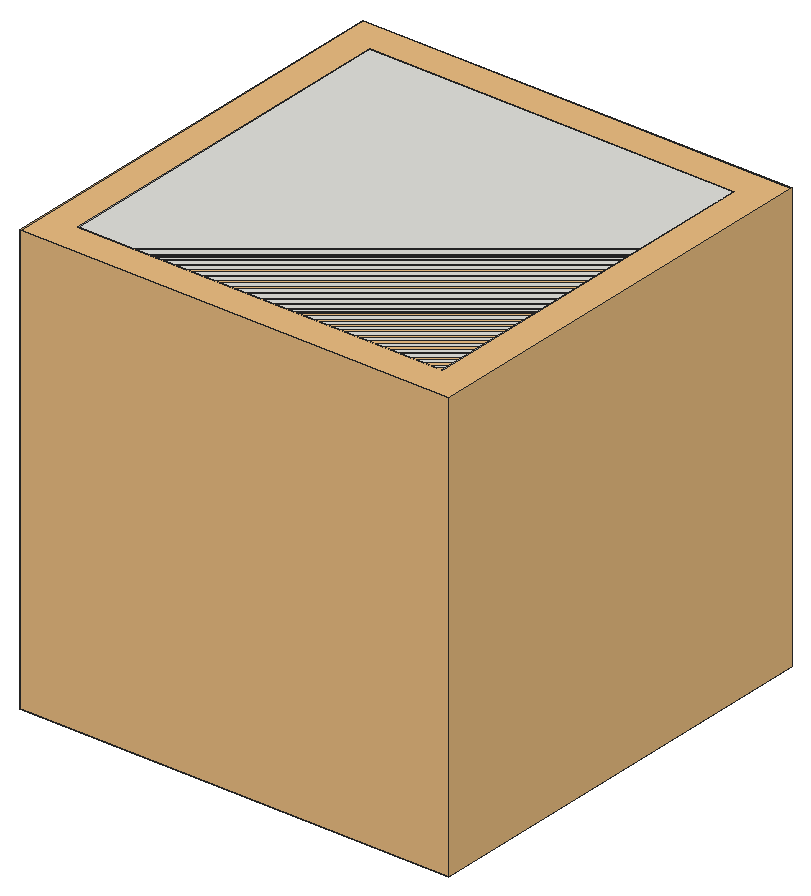
# SketchUp Ruby script. Lengths in inches.
U = 1.inch
M = Sketchup.active_model
def pt(a) = Geom::Point3d.new(a.map { |v| v * U })
def face(e, loops, mat)
  f = e.add_face(loops[0].map { |a| pt(a) })
  loops[1..].each { |l| e.add_face(l.map { |a| pt(a) }).erase! }
  f.material = f.back_material = mat if mat
  f
end
# faces: each face lists its corners as indices into pts; further lists are holes
def faces(e, pts, list, mat = nil) = list.each { |f| face(e, (f[0].is_a?(Array) ? f : [f]).map { |l| l.map { |i| pts[i] } }, mat) }
# xy, xz, yz: faces in a plane at the given z, y or x. An outline is a flat list of corners, or four numbers for a rectangle; further outlines are holes
def ring(l) = l.size == 4 ? [[l[0], l[1]], [l[2], l[1]], [l[2], l[3]], [l[0], l[3]]] : l.each_slice(2).to_a
def flat(e, list, mat, &to3) = list.each { |f| face(e, (f[0].is_a?(Array) ? f : [f]).map { |l| ring(l).map { |u, v| to3.(u, v) } }, mat) }
def xy(e, z, list, mat = nil) = flat(e, list, mat) { |x, y| [x, y, z] }
def xz(e, y, list, mat = nil) = flat(e, list, mat) { |x, z| [x, y, z] }
def yz(e, x, list, mat = nil) = flat(e, list, mat) { |y, z| [x, y, z] }
def lines(e, pts, list) = list.each { |a, b| e.add_line(pt(pts[a]), pt(pts[b])) }
# prism: a flat outline (further loops are holes) pulled along v
def prism(e, loops, v, mat = nil)
  f = face(e, loops, mat); d = Geom::Vector3d.new(v.map { |x| x * U })
  f.pushpull(f.normal.samedirection?(d) ? d.length : -d.length)
end
def box(e, o, s, mat = nil) = prism(e, [[o, [o[0] + s[0], o[1], o[2]], [o[0] + s[0], o[1] + s[1], o[2]], [o[0], o[1] + s[1], o[2]]]], [0, 0, s[2]], mat)
def at(x, y, z, deg = 0) = Geom::Transformation.translation(pt([x, y, z])) * Geom::Transformation.rotation(ORIGIN, Z_AXIS, deg.degrees)
def axes(o, x, y, z) = Geom::Transformation.new([*x, 0, *y, 0, *z, 0, *pt(o).to_a, 1])
def part(name) = M.definitions.add(name)
# library, detail: a bought-in or finely detailed component or shape, given as its bounding box
def library(name, o, s) = part(name).tap { |d| box(d.entities, o, s) }
def detail(e, o, s) = box(e.add_group.entities, o, s)
def put(e, d, t, mat = nil) = e.add_instance(d, t).tap { |i| i.material = mat if mat }
def group(e, t, mat = nil) = e.add_group.tap { |g| g.transformation = t; g.material = mat if mat }.entities
root = M.entities
M.materials.add("Pomeli-edt-511x511").color = [242, 209, 211]
M.materials.add("profumo-muschio-natures-511x511").color = [223, 234, 229]
c1 = library("Round ottoman",[0,0,0],[24.18,24.17,17.98])
c2 = library("Decoração+Banheiro",[28.69,-29.77,58.91],[5.39,6.58,5.91])
c3 = library("skpA613",[-33.11,-37.89,-86.79],[66.22,75.78,173.58])
c4 = library("Potted plant",[0.24,-1.94,0],[14.49,14.49,6.23])
c5 = library("ADORNOS+-+RMLLR",[6.19,-1.3125,-0.22],[15.35,11.9,12.07])
c6 = library("Toiletry bottle \#2",[0,0,0],[4.22,2.62,10.91])
c7 = library("Toiletry bottle \#3",[0,0,0],[4.22,2.62,10.91])
c8 = library("Toiletry bottle",[0,0,0],[3.45,3.45,11.12])
c9 = part("Component\#12")
xy(c9.entities,0,[[0,0,3.21,3.15]],"profumo-muschio-natures-511x511")
xy(c9.entities,9.32,[[0,0,3.21,3.15]])
xz(c9.entities,0,[[0,0,3.21,9.32]],"profumo-muschio-natures-511x511")
xz(c9.entities,3.15,[[0,0,3.21,9.32]])
yz(c9.entities,0,[[0,0,3.15,9.32]])
yz(c9.entities,3.21,[[0,0,3.15,9.32]])
c10 = library("Toiletry bottle \#1",[0,0,0],[3.45,3.45,11.12])
c11 = part("Component\#17")
xy(c11.entities,0,[[0,0,3.21,3.15]],"profumo-muschio-natures-511x511")
xy(c11.entities,9.32,[[0,0,3.21,3.15]])
xz(c11.entities,0,[[0,0,3.21,9.32]],"Pomeli-edt-511x511")
xz(c11.entities,3.15,[[0,0,3.21,9.32]])
yz(c11.entities,0,[[0,0,3.15,9.32]])
yz(c11.entities,3.21,[[0,0,3.15,9.32]])
c12 = library("Plant",[-15.17,-14.95,0],[35.27,31.45,46.14])
c13 = library("FILE+KEEPER",[308.125,87.4375,-0.08],[14,9.09,13.53])
c14 = library("Abstract sculpture",[0,0.06,0],[4.875,4.76,11.74])
c15 = library("Man+sculpture",[-5.14,-9.4,0],[7.87,19.56,27.58])
c16 = library("Group\#6",[0,0,0],[23.16,7,38.98])
c17 = library("Group\#5",[0,0,0],[23.16,7,38.98])
p = [[9,42.4,38],[9,42.4,39.47],[9,90.73,52.9],[9,90.73,52.9],[9,90.73,92.5],[9,90.73,92.5],
  [9,90.73,66.1],[9,90.73,66.1],[9,90.73,79.3],[9,90.73,79.3],[9,42.4,57.58],[9,42.4,106.96],
  [7.875,42.4,39.47],[9,18.02,39.47],[8.9375,18.02,39.47],[10,88.73,25.62],[21,88.73,25.62],[10,90.73,25.62],
  [21,90.73,25.62]]
lines(root,p,[[0,1],[2,3],[4,5],[6,7],[8,9],[10,11],[1,12],[13,14],[15,16],[17,18]])
detail(root,[0,0,0],[120,120,120])
put(root,c1,at(11.49,47.78,2))
put(root,c2,axes([-13.4,59.45,-37.71],[1,0,0],[0,1.12,0],[0,0,1.31]))
put(root,c3,axes([18.73,22.36,48.83],[0.1,0,0],[0,0.1,0],[0,0,0.1]))
put(root,c4,axes([12.39,97.06,93.1],[0.66461,0,0],[0,0.66461,0],[0,0,0.77354]))
put(root,c5,axes([19.38,89.3,80.39],[0,0.76608,0],[-0.672,0,0],[0,0,0.672]))
put(root,c6,at(20.1875,67,39.47,90))
put(root,c7,at(20.1875,71.22,39.47,90))
put(root,c8,axes([20.1875,64.61,39.47],[0,0.69,0],[-0.69,0,0],[0,0,0.85643]))
put(root,c9,axes([19.44,60.38,39.47],[0.12596,1.12296,0],[-1.12296,0.12596,0],[0,0,1.13]))
put(root,c10,axes([20.1875,75.4375,39.47],[0,0.69,0],[-0.69,0,0],[0,0,0.85643]))
put(root,c11,axes([20.1875,77.82,39.47],[0,1.13,0],[-1.13,0,0],[0,0,1.13]))
put(root,c12,axes([14.3,96.27,53.5],[0.22445,0,0],[0,0.22445,0],[0,0,0.22445]))
put(root,c13,axes([-39.39,290.18,40.01],[0,-0.61622,0],[0.61622,0,0],[0,0,0.61622]))
put(root,c14,at(14.41,103.55,40,-23.8))
put(root,c15,axes([14.47,102.92,53.5],[0.31,0,0],[0,0.31,0],[0,0,0.31]))
put(root,c16,axes([17.25,94.01,66.57],[0,0.20584,0],[-0.25731,0,0],[0,0,0.20584]))
put(root,c17,axes([17.25,100.44,66.57],[0,0.20584,0],[-0.25731,0,0],[0,0,0.20584]))
g1 = group(root,at(9,9,120))
xy(g1,-12,[[[0,0,102,102],[24,24,78,78]],[28,28,74,74]])
xy(g1,-11.5,[[[0,0,102,102],[23,23,79,79]],[23,23,24,78],[24,23,79,24],[78,24,79,78],[23,78,79,79]])
xy(g1,-11,[[[0,0,102,102],[23,23,79,79]],[[23,23,79,79],[28,28,74,74]]])
xy(g1,0,[[0,0,102,102]])
xz(g1,0,[[0,-12,102,-11.5],[0,-11.5,102,-11],[0,-11,102,0]])
xz(g1,23,[[23,-11.5,79,-11]])
xz(g1,24,[[24,-12,78,-11.5]])
xz(g1,28,[[28,-12,74,-11]])
xz(g1,74,[[28,-12,74,-11]])
xz(g1,78,[[24,-12,78,-11.5]])
xz(g1,79,[[23,-11.5,79,-11]])
xz(g1,102,[[0,-12,102,-11.5],[0,-11.5,102,-11],[0,-11,102,0]])
yz(g1,0,[[0,-12,102,-11.5],[0,-11.5,102,-11],[0,-11,102,0]])
yz(g1,23,[[23,-11.5,79,-11]])
yz(g1,24,[[24,-12,78,-11.5]])
yz(g1,28,[[28,-12,74,-11]])
yz(g1,74,[[28,-12,74,-11]])
yz(g1,78,[[24,-12,78,-11.5]])
yz(g1,79,[[23,-11.5,79,-11]])
yz(g1,102,[[0,-12,102,-11.5],[0,-11.5,102,-11],[0,-11,102,0]])
